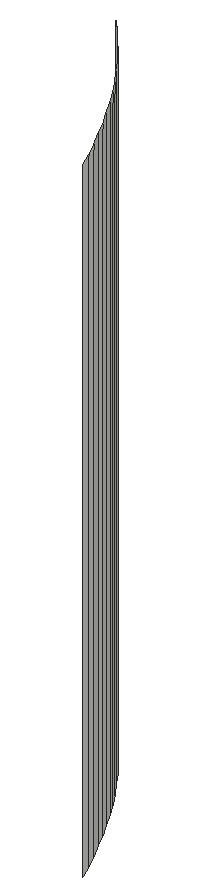
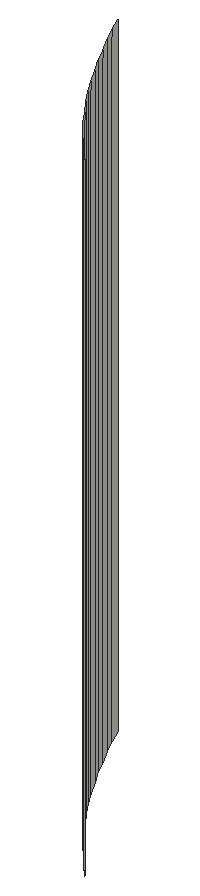
# SketchUp Ruby script. Lengths in inches.
U = 1.inch
M = Sketchup.active_model
def pt(a) = Geom::Point3d.new(a.map { |v| v * U })
def face(e, loops, mat)
  f = e.add_face(loops[0].map { |a| pt(a) })
  loops[1..].each { |l| e.add_face(l.map { |a| pt(a) }).erase! }
  f.material = f.back_material = mat if mat
  f
end
# faces: each face lists its corners as indices into pts; further lists are holes
def faces(e, pts, list, mat = nil) = list.each { |f| face(e, (f[0].is_a?(Array) ? f : [f]).map { |l| l.map { |i| pts[i] } }, mat) }
# xy, xz, yz: faces in a plane at the given z, y or x. An outline is a flat list of corners, or four numbers for a rectangle; further outlines are holes
def ring(l) = l.size == 4 ? [[l[0], l[1]], [l[2], l[1]], [l[2], l[3]], [l[0], l[3]]] : l.each_slice(2).to_a
def flat(e, list, mat, &to3) = list.each { |f| face(e, (f[0].is_a?(Array) ? f : [f]).map { |l| ring(l).map { |u, v| to3.(u, v) } }, mat) }
def xy(e, z, list, mat = nil) = flat(e, list, mat) { |x, y| [x, y, z] }
def xz(e, y, list, mat = nil) = flat(e, list, mat) { |x, z| [x, y, z] }
def yz(e, x, list, mat = nil) = flat(e, list, mat) { |y, z| [x, y, z] }
def lines(e, pts, list) = list.each { |a, b| e.add_line(pt(pts[a]), pt(pts[b])) }
# prism: a flat outline (further loops are holes) pulled along v
def prism(e, loops, v, mat = nil)
  f = face(e, loops, mat); d = Geom::Vector3d.new(v.map { |x| x * U })
  f.pushpull(f.normal.samedirection?(d) ? d.length : -d.length)
end
def box(e, o, s, mat = nil) = prism(e, [[o, [o[0] + s[0], o[1], o[2]], [o[0] + s[0], o[1] + s[1], o[2]], [o[0], o[1] + s[1], o[2]]]], [0, 0, s[2]], mat)
def at(x, y, z, deg = 0) = Geom::Transformation.translation(pt([x, y, z])) * Geom::Transformation.rotation(ORIGIN, Z_AXIS, deg.degrees)
def axes(o, x, y, z) = Geom::Transformation.new([*x, 0, *y, 0, *z, 0, *pt(o).to_a, 1])
def part(name) = M.definitions.add(name)
# library, detail: a bought-in or finely detailed component or shape, given as its bounding box
def library(name, o, s) = part(name).tap { |d| box(d.entities, o, s) }
def detail(e, o, s) = box(e.add_group.entities, o, s)
def put(e, d, t, mat = nil) = e.add_instance(d, t).tap { |i| i.material = mat if mat }
def group(e, t, mat = nil) = e.add_group.tap { |g| g.transformation = t; g.material = mat if mat }.entities
root = M.entities
p = [[326.76,321.18,231],[326.79,321.11,231],[326.79,321.11,234],[326.76,321.18,234],[326.73,321.25,231],[326.73,321.25,234],
  [326.69,321.32,231],[326.69,321.32,234],[326.66,321.39,231],[326.66,321.39,234],[326.62,321.46,231],[326.62,321.46,234],
  [326.54,321.6,231],[326.58,321.53,231],[326.58,321.53,234],[326.54,321.6,234],[326.5,321.66,231],[326.5,321.66,234],
  [326.41,321.79,231],[326.45,321.73,231],[326.45,321.73,234],[326.41,321.79,234],[326.36,321.85,231],[326.36,321.85,234],
  [326.31,321.91,231],[326.31,321.91,234],[326.26,321.97,231],[326.26,321.97,234],[326.21,322.03,231],[326.21,322.03,234]]
faces(root,p,[[0,1,2,3],[4,0,3,5],[6,4,5,7],[8,6,7,9],[10,8,9,11],[12,13,14,15],[13,10,11,14],[16,12,15,17],
  [18,19,20,21],[19,16,17,20],[22,18,21,23],[24,22,23,25],[26,24,25,27],[28,26,27,29]])
